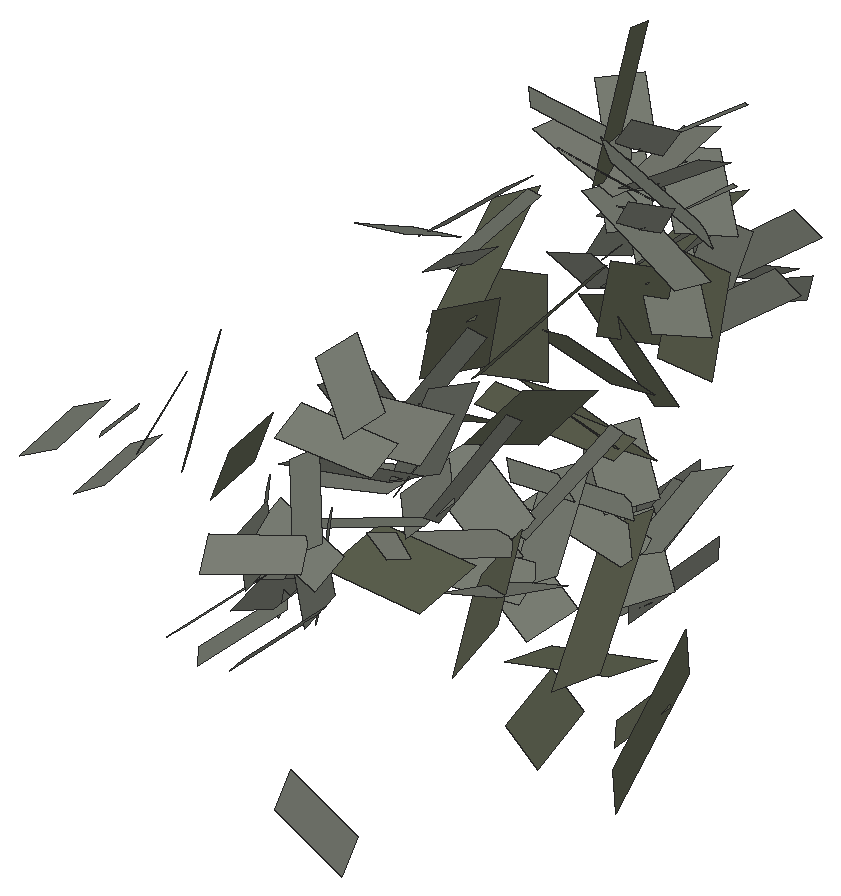
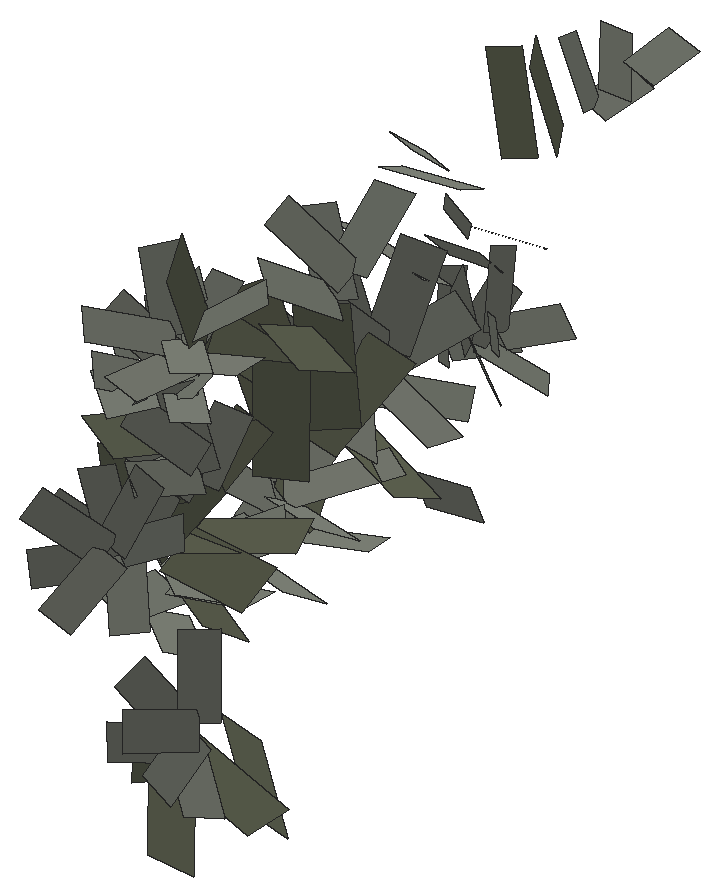
# SketchUp Ruby script. Lengths in inches.
U = 1.inch
M = Sketchup.active_model
def pt(a) = Geom::Point3d.new(a.map { |v| v * U })
def face(e, loops, mat)
  f = e.add_face(loops[0].map { |a| pt(a) })
  loops[1..].each { |l| e.add_face(l.map { |a| pt(a) }).erase! }
  f.material = f.back_material = mat if mat
  f
end
# faces: each face lists its corners as indices into pts; further lists are holes
def faces(e, pts, list, mat = nil) = list.each { |f| face(e, (f[0].is_a?(Array) ? f : [f]).map { |l| l.map { |i| pts[i] } }, mat) }
# xy, xz, yz: faces in a plane at the given z, y or x. An outline is a flat list of corners, or four numbers for a rectangle; further outlines are holes
def ring(l) = l.size == 4 ? [[l[0], l[1]], [l[2], l[1]], [l[2], l[3]], [l[0], l[3]]] : l.each_slice(2).to_a
def flat(e, list, mat, &to3) = list.each { |f| face(e, (f[0].is_a?(Array) ? f : [f]).map { |l| ring(l).map { |u, v| to3.(u, v) } }, mat) }
def xy(e, z, list, mat = nil) = flat(e, list, mat) { |x, y| [x, y, z] }
def xz(e, y, list, mat = nil) = flat(e, list, mat) { |x, z| [x, y, z] }
def yz(e, x, list, mat = nil) = flat(e, list, mat) { |y, z| [x, y, z] }
def lines(e, pts, list) = list.each { |a, b| e.add_line(pt(pts[a]), pt(pts[b])) }
# prism: a flat outline (further loops are holes) pulled along v
def prism(e, loops, v, mat = nil)
  f = face(e, loops, mat); d = Geom::Vector3d.new(v.map { |x| x * U })
  f.pushpull(f.normal.samedirection?(d) ? d.length : -d.length)
end
def box(e, o, s, mat = nil) = prism(e, [[o, [o[0] + s[0], o[1], o[2]], [o[0] + s[0], o[1] + s[1], o[2]], [o[0], o[1] + s[1], o[2]]]], [0, 0, s[2]], mat)
def at(x, y, z, deg = 0) = Geom::Transformation.translation(pt([x, y, z])) * Geom::Transformation.rotation(ORIGIN, Z_AXIS, deg.degrees)
def axes(o, x, y, z) = Geom::Transformation.new([*x, 0, *y, 0, *z, 0, *pt(o).to_a, 1])
def part(name) = M.definitions.add(name)
# library, detail: a bought-in or finely detailed component or shape, given as its bounding box
def library(name, o, s) = part(name).tap { |d| box(d.entities, o, s) }
def detail(e, o, s) = box(e.add_group.entities, o, s)
def put(e, d, t, mat = nil) = e.add_instance(d, t).tap { |i| i.material = mat if mat }
def group(e, t, mat = nil) = e.add_group.tap { |g| g.transformation = t; g.material = mat if mat }.entities
root = M.entities
M.materials.add("viburnumblaasdfas0df1w06d").color = [98, 102, 84]
M.materials.add("viburnumbladsadfasdfad0w122").color = [125, 129, 119]
c1 = part("Component\#315")
p = [[0.25,0,0],[2.05,0.01,0.35],[1.81,4.2,1.66],[0,4.19,1.3125]]
faces(c1.entities,p,[[0,1,2,3]],"viburnumbladsadfasdfad0w122")
c2 = part("viburnumblad2")
put(c2.entities,c1,axes([-19.23,-4.49,-32.18],[83.35428,0,0],[0,79.38502,0],[0,0,83.35428]))
c3 = part("Component\#314")
p = [[0.14,0,0],[2.58,0.05,0.25],[2.44,5.11,2.64],[0,5.05,2.39]]
faces(c3.entities,p,[[0,1,2,3]],"viburnumblaasdfas0df1w06d")
c4 = part("viburnumblad1\#2")
put(c4.entities,c3,axes([-37.25,6.23,19.31],[75.98784,0,0],[0,65.50676,0],[0,0,75.98784]))
put(root,c2,axes([1216.43,215.13,11.74],[-0.00707,-0.00889,-0.00124],[0.00366,-0.00429,0.00994],[-0.0082,0.00576,0.0055]))
put(root,c2,axes([1216.59,185.68,29.79],[-0.00855,-0.00051,-0.00592],[0.00282,-0.00961,-0.00317],[-0.00532,-0.00402,0.00702]))
put(root,c4,axes([1216.18,204.52,23.6],[0.01245,-0.00088,0.00582],[0.00019,0.01586,0.00199],[-0.00575,-0.00142,0.01169]))
put(root,c2,axes([1218.17,199.05,20.99],[0.00306,0.01272,-0.00021],[-0.01084,0.00248,-0.00806],[-0.00742,0.00196,0.01059]))
put(root,c2,axes([1218.14,217.13,20.99],[-0.00494,0.0045,-0.00826],[-0.00853,-0.00405,0.00272],[-0.002,0.0084,0.00497]))
put(root,c2,axes([1215.99,213.51,9.9375],[0.00828,0.00278,0.00738],[0.00071,0.00951,-0.00438],[-0.00785,0.00396,0.00731]))
put(root,c2,axes([1216.74,217.07,20.41],[0.00898,0.00541,-0.00233],[-0.00533,0.00547,-0.00762],[-0.00249,0.00719,0.00626]))
put(root,c2,axes([1216.97,212.625,9.47],[0.00739,0.00929,0.00129],[-0.00498,0.005,-0.00749],[-0.00707,0.00455,0.00775]))
put(root,c2,axes([1215.44,215,10.7],[0.00463,-0.00496,0.0092],[0.00608,0.00946,0.00204],[-0.0085,0.00407,0.00647]))
put(root,c4,axes([1219.13,211.04,8.24],[0.0024,0.01209,-0.00232],[-0.01101,0.00036,-0.0095],[-0.00784,0.00332,0.00921]))
put(root,c2,axes([1218.25,211.73,27.1875],[0.00073,0.01102,-0.00295],[-0.01141,0.00071,-0.00016],[0.00003,0.00295,0.01104]))
put(root,c2,axes([1217.31,212.5,28.37],[0.00853,0.00755,-0.00102],[-0.0076,0.00835,-0.00179],[-0.00044,0.00202,0.01125]))
put(root,c4,axes([1217.19,208.85,20.08],[-0.01129,-0.00613,-0.00067],[0.00417,-0.00777,0.01127],[-0.0047,0.00912,0.00614]))
put(root,c2,axes([1216.87,193.35,19.14],[0.0062,-0.00344,0.00762],[-0.00192,0.00879,0.00527],[-0.00787,-0.00449,0.00364]))
put(root,c2,axes([1217.29,204.44,28.46],[-0.01197,-0.00238,-0.00293],[0.00194,-0.01232,0.00219],[-0.00304,0.00182,0.01144]))
put(root,c2,axes([1215.57,214.4,22.54],[0.00794,-0.00459,0.00546],[0.00496,0.0095,0.00066],[-0.00518,0.00191,0.00818]))
put(root,c2,axes([1218.7,212.22,28.625],[-0.00749,0.00804,-0.00315],[-0.00863,-0.00712,0.00235],[-0.00031,0.00392,0.01074]))
put(root,c2,axes([1218.11,218.52,21.4],[-0.00984,-0.00064,-0.00419],[-0.00322,-0.006,0.00808],[-0.00275,0.0086,0.00434]))
put(root,c2,axes([1217.54,213.58,22.41],[-0.00996,-0.0034,-0.00378],[0.00101,-0.00837,0.00457],[-0.00471,0.00422,0.00764]))
put(root,c4,axes([1219.55,210.57,17.45],[0.00188,0.00994,-0.00772],[-0.0143,-0.00023,-0.00375],[-0.00243,0.00751,0.00854]))
put(root,c4,axes([1216.47,206.57,21.37],[-0.00729,-0.01049,-0.00199],[0.00959,-0.00792,0.00787],[-0.00649,0.00328,0.00895]))
put(root,c4,axes([1219.89,210.12,17.47],[-0.00372,0.0118,-0.00306],[-0.01362,-0.00502,-0.00283],[-0.00309,0.00191,0.01102]))
put(root,c4,axes([1219.18,207.09,6.59],[0.00499,0.00892,0.00903],[-0.00667,0.01209,-0.00778],[-0.01141,-0.0013,0.00685]))
put(root,c4,axes([1218.17,205.56,20.29],[-0.01203,-0.00093,-0.00471],[0.00029,-0.01476,0.00205],[-0.00435,0.00215,0.01023]))
put(root,c2,axes([1215.65,215.29,23.74],[0.00169,-0.00975,0.0041],[0.00892,0.0036,0.00459],[-0.00566,0.00263,0.0077]))
put(root,c2,axes([1218.57,203.94,16.51],[0.00718,0.01175,0.00394],[-0.01195,0.00776,-0.0014],[-0.003,-0.00258,0.01303]))
put(root,c2,axes([1218.125,193.01,18.45],[0.00371,0.00412,0.00878],[-0.006,0.0085,-0.00147],[-0.00737,-0.00446,0.00446]))
put(root,c2,axes([1218,211.73,25.68],[0.00819,0.00724,-0.00098],[-0.00821,0.00902,-0.00193],[-0.00044,0.00202,0.01125]))
put(root,c2,axes([1217.99,192.47,20.33],[-0.0062,0.00344,-0.00762],[-0.00004,-0.00961,-0.00424],[-0.0081,-0.00223,0.0048]))
put(root,c2,axes([1216.67,214.67,22.97],[-0.00555,-0.00919,0.00035],[0.0077,-0.00439,0.00674],[-0.00547,0.00359,0.00747]))
put(root,c2,axes([1215.85,205.11,26.62],[0.01052,-0.00734,0.00272],[0.00582,0.00933,0.00265],[-0.0036,-0.00095,0.01134]))
put(root,c2,axes([1216.47,218.62,20.44],[0.00984,0.00064,0.00419],[0.00246,0.0079,-0.00679],[-0.00344,0.00689,0.00616]))
put(root,c2,axes([1218.71,216.48,20.15],[-0.01027,-0.00067,-0.00437],[-0.0029,-0.0054,0.00727],[-0.00275,0.0086,0.00434]))
put(root,c2,axes([1216.76,187.05,29.11],[-0.0036,-0.00676,-0.00701],[0.00718,-0.00608,0.00197],[-0.00593,-0.00439,0.00637]))
put(root,c2,axes([1219.82,199.08,20.31],[-0.00427,0.01006,-0.00619],[-0.01054,-0.00775,-0.00533],[-0.00749,0.00313,0.01026]))
put(root,c2,axes([1218.93,192.4,19.32],[-0.00506,0.00898,-0.002],[-0.00471,-0.00455,-0.00828],[-0.00753,-0.00286,0.00529]))
put(root,c2,axes([1217.82,186.96,28.28],[-0.00729,-0.00007,-0.00611],[0.00282,-0.00961,-0.00317],[-0.00621,-0.00405,0.00634]))
put(root,c2,axes([1215.875,205.43,28.0625],[0.00228,-0.01232,0.00076],[0.0106,0.00221,0.00397],[-0.00422,0.00003,0.01117]))
put(root,c2,axes([1219.18,199.8,21.77],[-0.00935,0.0021,-0.00891],[-0.00409,-0.01235,0.00138],[-0.00819,0.00377,0.00948]))
put(root,c2,axes([1220.17,203.87,15.21],[-0.00305,0.01398,0.00068],[-0.01364,-0.00282,-0.0033],[-0.00279,-0.00128,0.01326]))
put(root,c4,axes([1217.56,212.57,26.51],[0.00608,-0.01136,0.00423],[0.00607,0.0078,0.01224],[-0.01094,-0.0031,0.0074]))
put(root,c2,axes([1216.96,214.77,10.13],[-0.00173,-0.0098,0.00563],[0.00735,0.00343,0.00822],[-0.00865,0.00481,0.00572]))
put(root,c2,axes([1218.14,200.79,22.87],[-0.00877,-0.00751,-0.00615],[0.00336,-0.01013,0.00757],[-0.0091,0.00349,0.00872]))
put(root,c2,axes([1217.44,193.67,20.27],[0.00095,-0.00927,-0.00479],[0.00517,-0.00382,0.00808],[-0.00874,-0.00294,0.00329]))
put(root,c2,axes([1216.61,214.25,21.69],[0.00162,-0.00936,0.00394],[0.00963,0.00389,0.00496],[-0.00566,0.00263,0.0077]))
put(root,c4,axes([1220.125,212.78,18.4],[-0.00938,0.00386,-0.00599],[-0.00819,-0.00718,0.008],[-0.00057,0.00892,0.00623]))
put(root,c4,axes([1221.02,198.39,17.1],[0.00387,0.01311,0.00437],[-0.0121,0.00667,-0.00928],[-0.00906,-0.00102,0.01108]))
put(root,c2,axes([1217.14,205.2,27.03],[-0.00587,-0.00963,-0.00252],[0.00967,-0.00694,0.00401],[-0.00471,0.00005,0.01098]))
put(root,c2,axes([1220.28,203.97,17.1],[-0.01149,0.00801,-0.00297],[-0.00766,-0.01186,-0.00235],[-0.00352,-0.00017,0.01315]))
put(root,c2,axes([1218.64,199.49,19.21],[0.00916,0.00784,0.00642],[-0.00492,0.00961,-0.00471],[-0.00802,0.00094,0.01029]))
put(root,c2,axes([1217.57,200.21,20.17],[0.00935,-0.0021,0.00891],[0.00182,0.01184,0.00088],[-0.00893,0.00067,0.00953]))
put(root,c2,axes([1217,187.74,28.18],[0.0036,-0.00945,-0.00418],[0.00709,-0.00011,0.00601],[-0.00594,-0.00519,0.00581]))
put(root,c2,axes([1217.04,201.33,21.75],[0.00445,-0.01048,0.00645],[0.00766,0.00772,0.00727],[-0.00963,0.0013,0.00876]))
put(root,c2,axes([1217.21,213.75,9.01],[0.00508,-0.00494,0.00777],[0.00608,0.00946,0.00204],[-0.00795,0.00351,0.00743]))
put(root,c2,axes([1217.5,212.7,26.8],[0.01133,-0.00035,0.0015],[0.00059,0.01187,-0.00167],[-0.00144,0.00165,0.01122]))
put(root,c4,axes([1219.79,211.83,19.22],[-0.0112,0.0013,-0.00343],[-0.00292,-0.0124,0.00476],[-0.00244,0.00473,0.0094]))
put(root,c4,axes([1217.81,189.04,26.23],[0.00672,-0.00928,0.00091],[0.00601,0.00561,0.01016],[-0.00772,-0.00461,0.00599]))
put(root,c2,axes([1220.09,204.41,13.46],[0.00689,0.01128,0.00378],[-0.0129,0.00838,-0.00151],[-0.003,-0.00258,0.01303]))
put(root,c2,axes([1218.38,217.96,20.08],[-0.00898,-0.00541,0.00233],[0.00475,-0.00369,0.00928],[-0.0037,0.00829,0.00425]))
put(root,c4,axes([1219.84,210.46,6.09],[0.00721,0.00805,0.00636],[-0.00379,0.01064,-0.00917],[-0.00973,0.00288,0.00737]))
put(root,c2,axes([1219.48,212.53,27.11],[-0.01133,0.00035,-0.0015],[-0.0009,-0.01068,0.0043],[-0.00126,0.00434,0.0105]))
put(root,c2,axes([1219.45,209.67,15.99],[0.00933,0.00906,0.00093],[-0.00886,0.00934,-0.00204],[-0.00208,0.00083,0.01284]))
put(root,c2,axes([1218.1,194.03,19.05],[0.00506,-0.00898,0.002],[0.00284,0.00386,0.00969],[-0.00844,-0.00386,0.00315]))
put(root,c2,axes([1220.73,208.99,14.6875],[0.00055,0.01289,-0.00188],[-0.01292,0.00032,-0.00165],[-0.00158,0.00193,0.01279]))
put(root,c2,axes([1219.04,193.92,18.125],[0.00595,-0.0033,0.00732],[-0.00208,0.00949,0.0057],[-0.00787,-0.00449,0.00364]))
put(root,c2,axes([1221.01,209.38,16.42],[-0.00854,0.00917,-0.00359],[-0.00964,-0.00875,0.0006],[-0.00199,0.00305,0.01252]))
put(root,c4,axes([1218.62,213.3,20.15],[-0.00897,-0.00759,0.00065],[0.00732,-0.00776,0.00825],[-0.00418,0.00599,0.00812]))
put(root,c2,axes([1217.29,217.97,19.55],[0.00494,-0.0045,0.00826],[0.00853,0.00632,-0.00167],[-0.00419,0.00708,0.00554]))
put(root,c2,axes([1218.82,193.72,19.99],[-0.00371,-0.00412,-0.00878],[0.00371,-0.00856,0.0023],[-0.0086,-0.00227,0.00398]))
put(root,c2,axes([1217.69,219.19,20.33],[-0.00286,-0.007,0.00749],[0.00939,0.00159,0.0048],[-0.00429,0.00766,0.00474]))
put(root,c4,axes([1217.16,205.7,21.68],[0.00673,-0.01108,0.00456],[0.01197,0.00933,0.00501],[-0.00603,0.0015,0.01157]))
put(root,c4,axes([1218.1,212.01,22.64],[0.01125,-0.00276,0.00479],[0.00395,0.01395,-0.00123],[-0.00436,0.00225,0.01154]))
put(root,c2,axes([1218.95,204.89,14.89],[0.0132,0.00264,0.00489],[-0.00375,0.01436,0.00234],[-0.00402,-0.00331,0.01259]))
put(root,c2,axes([1221.58,211.2,24.96],[-0.00115,0.01298,-0.0064],[-0.01441,0.00008,0.00199],[0.00223,0.00688,0.01234]))
put(root,c4,axes([1219.66,214.86,18.45],[-0.01138,-0.00264,0.00129],[0.00289,-0.0057,0.01174],[-0.00153,0.01008,0.00426]))
put(root,c2,axes([1219.97,193.29,19.41],[-0.00487,0.00336,-0.00745],[-0.00004,-0.00961,-0.00424],[-0.00872,-0.00185,0.00395]))
put(root,c2,axes([1217.64,213.87,28.04],[0.00749,-0.00804,0.00315],[0.0083,0.00786,0.00032],[-0.00239,0.00208,0.01099]))
put(root,c2,axes([1220.57,212.44,26.37],[0.0095,0.00972,-0.00486],[-0.01098,0.00941,-0.00264],[0.00181,0.00573,0.01291]))
put(root,c2,axes([1218.19,217.08,19.07],[-0.00274,-0.00672,0.00719],[0.01014,0.00172,0.00518],[-0.00429,0.00766,0.00474]))
put(root,c2,axes([1221.41,190.21,22.56],[-0.00345,0.00905,0.004],[-0.00954,-0.00184,-0.00399],[-0.00252,-0.00485,0.0079]))
put(root,c2,axes([1219.04,213.59,28.29],[-0.00853,-0.00755,0.00102],[0.00727,-0.00761,0.00446],[-0.00226,0.00398,0.01048]))
put(root,c2,axes([1218.79,201.27,21.0625],[-0.00306,-0.01272,0.00021],[0.00831,-0.00183,0.01011],[-0.0097,0.00247,0.00842]))
put(root,c2,axes([1220.63,209.16,12.96],[0.00895,0.00869,0.00089],[-0.00957,0.01008,-0.0022],[-0.00208,0.00083,0.01284]))
put(root,c2,axes([1220.91,210.74,23.23],[0.00912,0.00933,-0.00467],[-0.01186,0.01016,-0.00285],[0.00181,0.00573,0.01291]))
put(root,c2,axes([1222.02,195.87,24.8],[0.00095,0.01366,0.00535],[-0.01286,0.00336,-0.00628],[-0.00706,-0.00428,0.01216]))
put(root,c2,axes([1218.2,213.13,25.36],[0.00782,-0.00839,0.00329],[0.00747,0.00707,0.00029],[-0.00239,0.00208,0.01099]))
put(root,c2,axes([1218.43,213.66,26.64],[-0.00073,-0.01102,0.00295],[0.01017,0.00002,0.00259],[-0.00273,0.00304,0.01068]))
put(root,c2,axes([1219.39,212.97,25.64],[-0.00757,-0.0073,-0.00011],[0.00727,-0.00761,0.00446],[-0.00317,0.00314,0.01053]))
put(root,c2,axes([1221.35,191.07,21.51],[0.00404,0.00727,0.00631],[-0.0093,0.00487,0.00025],[-0.00255,-0.00567,0.00738]))
put(root,c2,axes([1219.54,194.33,19.27],[0.00099,-0.00968,-0.005],[0.00466,-0.00344,0.00728],[-0.00874,-0.00294,0.00329]))
put(root,c2,axes([1218.48,205.74,16.7],[0.01149,-0.00801,0.00297],[0.00658,0.01147,0.00547],[-0.00527,-0.00304,0.01219]))
put(root,c2,axes([1222.41,212.26,26.45],[-0.01112,0.00864,-0.0042],[-0.00937,-0.00881,0.00635],[0.00161,0.00797,0.01181]))
put(root,c2,axes([1220.39,191.06,22.61],[0.00916,0.00124,0.00492],[-0.00387,0.00837,0.00487],[-0.00322,-0.0061,0.00681]))
put(root,c2,axes([1219.03,200.84,19.375],[0.00502,-0.00971,0.00503],[0.00766,0.00772,0.00727],[-0.00909,0.00016,0.0094]))
put(root,c2,axes([1221.75,191.88,9.95],[0.00409,0.00375,0.00971],[-0.00938,0.00585,0.00169],[-0.00452,-0.00876,0.00528]))
put(root,c4,axes([1220.5625,206.04,10.22],[0.01357,-0.0015,0.0077],[-0.00069,0.01762,0.00453],[-0.00774,-0.0037,0.01228]))
put(root,c4,axes([1219.48,190.1875,25.78],[-0.00104,-0.01037,-0.00489],[0.01073,-0.00422,0.00645],[-0.0067,-0.00317,0.00766]))
put(root,c4,axes([1221.875,198.92,14.625],[0.00862,0.00382,0.01082],[-0.00301,0.01604,-0.00327],[-0.01117,-0.00026,0.009]))
put(root,c2,axes([1221.43,192.65,27.0625],[0.00759,0.00699,0.00431],[-0.00767,0.00813,0.00032],[-0.00293,-0.00317,0.01031]))
put(root,c2,axes([1219.86,210.1,14.27],[0.01264,-0.00008,0.0032],[0.00017,0.01368,-0.00036],[-0.00319,0.00037,0.01263]))
put(root,c4,axes([1221.28,208.28,4.89],[0.00484,-0.00571,0.01239],[0.00394,0.01587,0.00555],[-0.01361,0.00143,0.00513]))
put(root,c2,axes([1221.3,205.21,15.76],[-0.0132,-0.00264,-0.00489],[0.00251,-0.01421,0.00089],[-0.00477,0.0001,0.01275]))
put(root,c2,axes([1222.66,192.59,25.94],[0.00024,0.01092,0.00238],[-0.01143,0.00081,-0.00255],[-0.00254,-0.00227,0.01065]))
put(root,c4,axes([1219.29,205.7,19.66],[-0.0079,-0.01248,0.00117],[0.01398,-0.00821,0.00596],[-0.0035,0.004,0.01323]))
